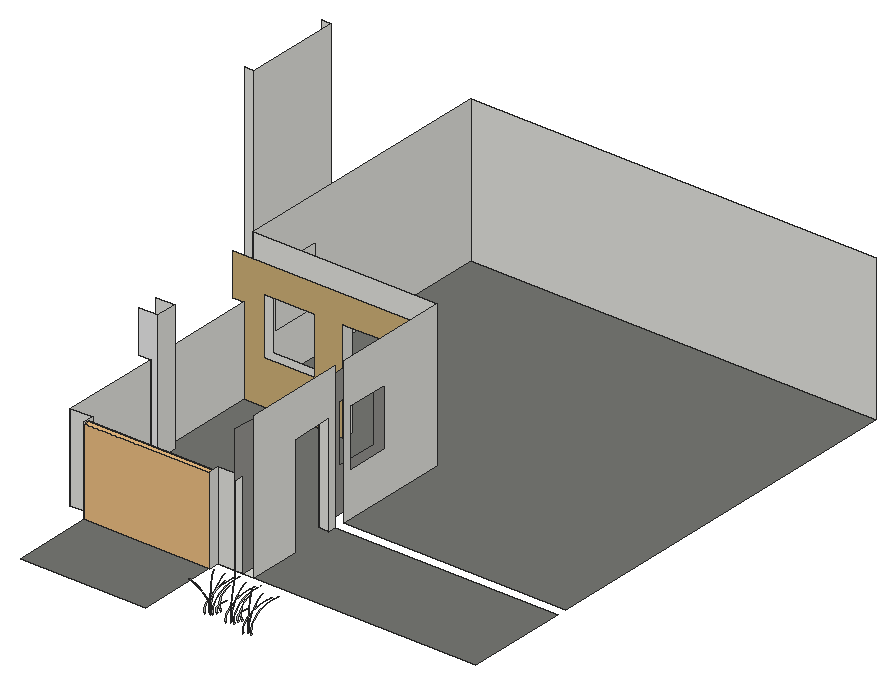
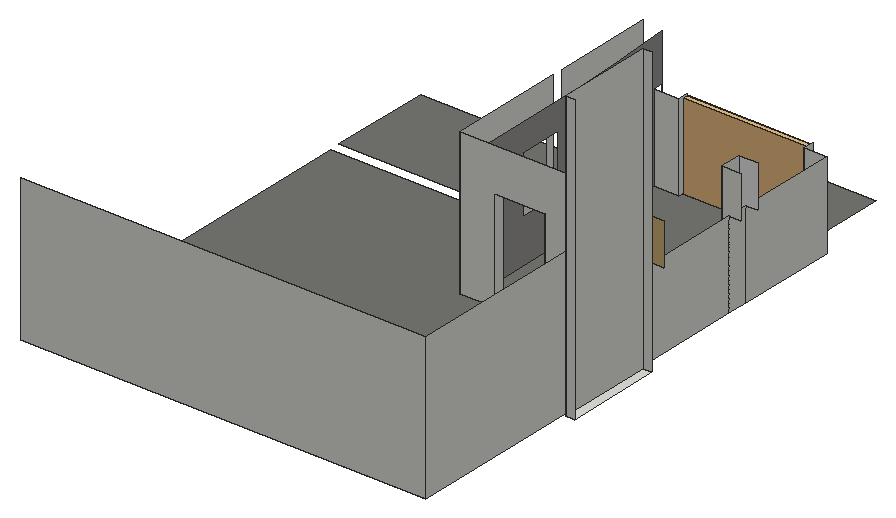
# SketchUp Ruby script. Lengths in inches.
U = 1.inch
M = Sketchup.active_model
def pt(a) = Geom::Point3d.new(a.map { |v| v * U })
def face(e, loops, mat)
  f = e.add_face(loops[0].map { |a| pt(a) })
  loops[1..].each { |l| e.add_face(l.map { |a| pt(a) }).erase! }
  f.material = f.back_material = mat if mat
  f
end
# faces: each face lists its corners as indices into pts; further lists are holes
def faces(e, pts, list, mat = nil) = list.each { |f| face(e, (f[0].is_a?(Array) ? f : [f]).map { |l| l.map { |i| pts[i] } }, mat) }
# xy, xz, yz: faces in a plane at the given z, y or x. An outline is a flat list of corners, or four numbers for a rectangle; further outlines are holes
def ring(l) = l.size == 4 ? [[l[0], l[1]], [l[2], l[1]], [l[2], l[3]], [l[0], l[3]]] : l.each_slice(2).to_a
def flat(e, list, mat, &to3) = list.each { |f| face(e, (f[0].is_a?(Array) ? f : [f]).map { |l| ring(l).map { |u, v| to3.(u, v) } }, mat) }
def xy(e, z, list, mat = nil) = flat(e, list, mat) { |x, y| [x, y, z] }
def xz(e, y, list, mat = nil) = flat(e, list, mat) { |x, z| [x, y, z] }
def yz(e, x, list, mat = nil) = flat(e, list, mat) { |y, z| [x, y, z] }
def lines(e, pts, list) = list.each { |a, b| e.add_line(pt(pts[a]), pt(pts[b])) }
# prism: a flat outline (further loops are holes) pulled along v
def prism(e, loops, v, mat = nil)
  f = face(e, loops, mat); d = Geom::Vector3d.new(v.map { |x| x * U })
  f.pushpull(f.normal.samedirection?(d) ? d.length : -d.length)
end
def box(e, o, s, mat = nil) = prism(e, [[o, [o[0] + s[0], o[1], o[2]], [o[0] + s[0], o[1] + s[1], o[2]], [o[0], o[1] + s[1], o[2]]]], [0, 0, s[2]], mat)
def at(x, y, z, deg = 0) = Geom::Transformation.translation(pt([x, y, z])) * Geom::Transformation.rotation(ORIGIN, Z_AXIS, deg.degrees)
def axes(o, x, y, z) = Geom::Transformation.new([*x, 0, *y, 0, *z, 0, *pt(o).to_a, 1])
def part(name) = M.definitions.add(name)
# library, detail: a bought-in or finely detailed component or shape, given as its bounding box
def library(name, o, s) = part(name).tap { |d| box(d.entities, o, s) }
def detail(e, o, s) = box(e.add_group.entities, o, s)
def put(e, d, t, mat = nil) = e.add_instance(d, t).tap { |i| i.material = mat if mat }
def group(e, t, mat = nil) = e.add_group.tap { |g| g.transformation = t; g.material = mat if mat }.entities
root = M.entities
M.materials.add("Metal_Seamed").color = [118, 119, 115]
M.materials.add("[Chipboard]").color = [205, 176, 119]
M.materials.add("[Granite Light Gray]").color = [149, 148, 144]
M.materials.add("white_wall").color = [233, 233, 233]
c1 = library("Merbau Gate Metal Frame",[0,0,0],[4.48,115.59,70.87])
xy(root,0,[[372.21,325.52,381.21,367.52],[229.21,408.6,235.21,426.23],[219.74,518.03,227.09,597.83]])
xy(root,0,[[247.49,251,351.06,251,351.06,317.12,351.48,317.12,351.48,325.52,372.21,325.52,372.21,367.52,381.21,367.52,381.21,325.52,565.21,325.52,565.21,409.52,381.21,409.52,381.21,403.52,372.21,403.52,372.21,505.52,352.83,505.52,352.83,514.52,381.21,514.52,381.21,418.52,565.21,418.52,565.21,739.58,229.21,739.58,229.21,514.52,310.83,514.52,310.83,505.52,229.21,505.52,229.21,426.23,235.21,426.23,235.21,408.6,229.21,408.6,229.21,325.52,247.49,325.52]],"Metal_Seamed")
xz(root,325.52,[[229.21,0,247.49,72],[351.48,0,372.21,72]])
xz(root,367.52,[[372.21,0,381.21,84]])
xz(root,403.52,[[372.21,0,381.21,84]])
xz(root,408.6,[[229.21,0,229.21,72,219.74,72,219.74,106.875,235.21,106.875,235.21,0]],"white_wall")
xz(root,426.23,[[229.21,0,235.21,0,235.21,106.875,219.74,106.875,219.74,72,229.21,72]])
xz(root,505.52,[[[229.21,0,310.83,0,310.83,84,352.83,84,352.83,0,372.21,0,372.21,106.875,219.74,106.875,219.74,72,229.21,72],[245.65,36,287.65,84]]],"[Chipboard]")
xz(root,514.52,[[[229.21,0,229.21,120,381.21,120,381.21,0,352.83,0,352.83,84,310.83,84,310.83,0],[245.65,36,287.65,84]]])
xz(root,518.03,[[219.74,0,227.09,237.3]])
xz(root,597.83,[[219.74,0,227.09,237.3]])
xz(root,739.58,[[229.21,0,565.21,120]])
yz(root,227.09,[[518.03,0,597.83,237.3]])
yz(root,229.21,[[325.52,0,408.6,72],[408.6,0,426.23,72],[426.23,0,505.52,72],[[514.52,0,739.58,120],[537.64,36,579.64,84]]])
yz(root,235.21,[[408.6,0,426.23,106.875]])
yz(root,247.49,[[317.12,0,325.52,72]])
yz(root,310.83,[[505.52,0,514.52,84]])
yz(root,351.48,[[317.12,0,325.52,72]])
yz(root,352.83,[[505.52,0,514.52,84]])
yz(root,372.21,[[317.12,0,317.13,0,317.13,72],[317.12,0,317.13,72,317.12,72],[[325.52,0,325.52,72,317.14,72,317.14,111,359.56,108.74,394.5,106.875,505.52,106.875,505.52,0,403.52,0,403.52,84,367.52,84,367.52,0],[424.52,36,460.52,84]]],"[Granite Light Gray]")
yz(root,381.21,[[325.52,0,367.52,0,367.52,84,403.52,84,403.52,0,409.52,0,409.52,120,325.52,120],[[418.52,0,514.52,120],[424.52,36,460.52,84]]])
g1 = group(root,at(386.9,271.43,0))
p = [[7.51,7.51,22.54],[6.3125,6.3125,20.88],[5.21,5.21,19.16],[4.21,4.21,17.39],[3.32,3.32,15.57],[2.52,2.52,13.71],
  [1.84,1.84,11.82],[1.27,1.27,9.89],[0.81,0.81,7.94],[0.46,0.46,5.97],[0.22,0.22,3.99],[0.1,0.1,2],
  [0.1,0.1,0],[0,0,2.01],[0.04,0.04,4.01],[0.21,0.21,6.01],[0.51,0.51,8],[0.95,0.95,9.97],
  [1.51,1.51,11.91],[2.21,2.21,13.81],[3.03,3.03,15.67],[3.98,3.98,17.48],[5.04,5.04,19.23],[6.22,6.22,20.92]]
faces(g1,p,[[0,1,2,3,4,5,6,7,8,9,10,11,12,13,14,15,16,17,18,19,20,21,22,23]])
g2 = group(root,at(390.32,270.24,0))
p = [[-0.93,0.35,0],[-0.41,0.16,0],[0,0,1.75],[-0.17,0.0625,3.51],[-0.91,0.34,5.24],[-2.21,0.83,6.89],
  [-4.03,1.52,8.42],[-6.34,2.39,9.8],[-9.0625,3.42,10.98],[-12.14,4.59,11.95],[-15.5,5.86,12.67],[-19.06,7.2,13.13],
  [-22.72,8.58,13.32],[-26.4,9.97,13.23],[-22.79,8.61,13.25],[-19.22,7.26,13],[-15.76,5.96,12.5],[-12.51,4.73,11.75],
  [-9.53,3.6,10.78],[-6.89,2.6,9.6],[-4.65,1.76,8.25],[-2.87,1.08,6.75],[-1.58,0.6,5.13],[-0.82,0.31,3.44],
  [-0.6,0.23,1.72]]
faces(g2,p,[[0,1,2,3,4,5,6,7,8,9,10,11,12,13,14,15,16,17,18,19,20,21,22,23,24]])
g3 = group(root,at(409.22,272.74,0))
p = [[5.08,5.08,9.0625],[4.15,4.15,8.49],[3.31,3.31,7.85],[2.57,2.57,7.18],[1.93,1.93,6.45],[1.41,1.41,5.7],
  [0.99,0.99,4.91],[0.7,0.7,4.1],[0.53,0.53,3.28],[0.48,0.48,2.45],[0.55,0.55,1.625],[0.75,0.75,0.8],
  [1.0625,1.0625,0],[0.65,0.65,0],[0.3,0.3,0.81],[0.08,0.08,1.65],[0,0,2.49],[0.06,0.06,3.34],
  [0.25,0.25,4.17],[0.58,0.58,4.99],[1.04,1.04,5.79],[1.62,1.62,6.54],[2.33,2.33,7.26],[3.14,3.14,7.92],
  [4.0625,4.0625,8.52]]
faces(g3,p,[[0,1,2,3,4,5,6,7,8,9,10,11,12,13,14,15,16,17,18,19,20,21,22,23,24]])
g4 = group(root,at(391.36,273.16,0))
p = [[5.08,5.08,9.0625],[4.15,4.15,8.49],[3.31,3.31,7.85],[2.57,2.57,7.18],[1.93,1.93,6.45],[1.41,1.41,5.7],
  [0.99,0.99,4.91],[0.7,0.7,4.1],[0.53,0.53,3.28],[0.48,0.48,2.45],[0.55,0.55,1.625],[0.75,0.75,0.8],
  [1.0625,1.0625,0],[0.65,0.65,0],[0.3,0.3,0.81],[0.08,0.08,1.65],[0,0,2.49],[0.06,0.06,3.34],
  [0.25,0.25,4.17],[0.58,0.58,4.99],[1.04,1.04,5.79],[1.62,1.62,6.54],[2.33,2.33,7.26],[3.14,3.14,7.92],
  [4.0625,4.0625,8.52]]
faces(g4,p,[[0,1,2,3,4,5,6,7,8,9,10,11,12,13,14,15,16,17,18,19,20,21,22,23,24]])
g5 = group(root,at(424.25,265.37,0))
p = [[-0.5,0.78,0],[-0.22,0.34,0],[0,0,2.37],[-0.09,0.14,4.75],[-0.49,0.76,7.08],[-1.2,1.84,9.32],
  [-2.1875,3.37,11.39],[-3.4375,5.29,13.25],[-4.92,7.57,14.85],[-6.59,10.14,16.15],[-8.41,12.95,17.13],[-10.34,15.92,17.75],
  [-12.32,18.97,18.01],[-14.32,22.05,17.89],[-12.36,19.03,17.91],[-10.42,16.05,17.58],[-8.55,13.16,16.9],[-6.78,10.45,15.89],
  [-5.17,7.96,14.58],[-3.73,5.75,12.99],[-2.52,3.88,11.15],[-1.55,2.39,9.125],[-0.86,1.32,6.94],[-0.44,0.68,4.66],
  [-0.33,0.5,2.33]]
faces(g5,p,[[0,1,2,3,4,5,6,7,8,9,10,11,12,13,14,15,16,17,18,19,20,21,22,23,24]])
g6 = group(root,at(421.55,263.18,0))
p = [[0.08,0.99,0],[0.03,0.44,0],[0,0,2.01],[0.01,0.18,4.04],[0.08,0.97,6.02],[0.19,2.35,7.92],
  [0.34,4.3,9.68],[0.53,6.75,11.26],[0.76,9.66,12.62],[1.02,12.94,13.73],[1.3,16.52,14.5625],[1.6,20.31,15.09],
  [1.91,24.21,15.31],[2.21,28.13,15.2],[1.91,24.29,15.22],[1.61,20.48,14.94],[1.32,16.8,14.37],[1.05,13.33,13.51],
  [0.8,10.15,12.39],[0.58,7.34,11.04],[0.39,4.95,9.48],[0.24,3.05,7.75],[0.13,1.68,5.9],[0.07,0.87,3.96],
  [0.05,0.64,1.98]]
faces(g6,p,[[0,1,2,3,4,5,6,7,8,9,10,11,12,13,14,15,16,17,18,19,20,21,22,23,24]])
g7 = group(root,at(427.01,264.89,0))
p = [[0.07,0.92,0],[0.03,0.41,0],[0,0,2.37],[0.01,0.17,4.75],[0.07,0.9,7.08],[0.17,2.19,9.32],
  [0.32,4,11.39],[0.5,6.29,13.25],[0.71,9,14.85],[0.95,12.06,16.15],[1.21,15.39,17.13],[1.49,18.92,17.75],
  [1.78,22.55,18.01],[2.0625,26.21,17.89],[1.78,22.625,17.91],[1.5,19.08,17.58],[1.23,15.65,16.9],[0.98,12.42,15.89],
  [0.74,9.46,14.58],[0.54,6.84,12.99],[0.36,4.61,11.15],[0.22,2.84,9.125],[0.125,1.57,6.94],[0.0625,0.8125,4.66],
  [0.05,0.59,2.33]]
faces(g7,p,[[0,1,2,3,4,5,6,7,8,9,10,11,12,13,14,15,16,17,18,19,20,21,22,23,24]])
g8 = group(root,at(409.57,275.82,0))
p = [[5.08,5.08,18.42],[4.15,4.15,17.25],[3.31,3.31,15.97],[2.57,2.57,14.59],[1.93,1.93,13.12],[1.41,1.41,11.58],
  [0.99,0.99,9.98],[0.7,0.7,8.34],[0.53,0.53,6.67],[0.48,0.48,4.99],[0.55,0.55,3.3],[0.75,0.75,1.63],
  [1.0625,1.0625,0],[0.65,0.65,0],[0.3,0.3,1.66],[0.08,0.08,3.35],[0,0,5.07],[0.06,0.06,6.79],
  [0.25,0.25,8.49],[0.58,0.58,10.15],[1.04,1.04,11.76],[1.62,1.62,13.3],[2.33,2.33,14.75],[3.14,3.14,16.1],
  [4.0625,4.0625,17.33]]
faces(g8,p,[[0,1,2,3,4,5,6,7,8,9,10,11,12,13,14,15,16,17,18,19,20,21,22,23,24]])
g9 = group(root,at(391.7,276.23,0))
p = [[5.08,5.08,18.42],[4.15,4.15,17.25],[3.31,3.31,15.97],[2.57,2.57,14.59],[1.93,1.93,13.12],[1.41,1.41,11.58],
  [0.99,0.99,9.98],[0.7,0.7,8.34],[0.53,0.53,6.67],[0.48,0.48,4.99],[0.55,0.55,3.3],[0.75,0.75,1.63],
  [1.0625,1.0625,0],[0.65,0.65,0],[0.3,0.3,1.66],[0.08,0.08,3.35],[0,0,5.07],[0.06,0.06,6.79],
  [0.25,0.25,8.49],[0.58,0.58,10.15],[1.04,1.04,11.76],[1.62,1.62,13.3],[2.33,2.33,14.75],[3.14,3.14,16.1],
  [4.0625,4.0625,17.33]]
faces(g9,p,[[0,1,2,3,4,5,6,7,8,9,10,11,12,13,14,15,16,17,18,19,20,21,22,23,24]])
g10 = group(root,at(423.97,266.21,0))
p = [[-0.27,0.88,0],[-0.12,0.39,0],[0,0,2.0625],[-0.05,0.16,4.13],[-0.26,0.87,6.16],[-0.64,2.1,8.1],
  [-1.17,3.84,9.91],[-1.84,6.03,11.52],[-2.64,8.63,12.92],[-3.54,11.5625,14.05],[-4.51,14.76,14.9],[-5.55,18.15,15.45],
  [-6.61,21.64,15.67],[-7.69,25.14,15.5625],[-6.63,21.7,15.58],[-5.59,18.3,15.29],[-4.59,15.01,14.71],[-3.64,11.91,13.83],
  [-2.77,9.07,12.68],[-2,6.56,11.3],[-1.35,4.43,9.7],[-0.83,2.73,7.9375],[-0.46,1.5,6.04],[-0.24,0.78,4.05],
  [-0.17,0.57,2.02]]
faces(g10,p,[[0,1,2,3,4,5,6,7,8,9,10,11,12,13,14,15,16,17,18,19,20,21,22,23,24]])
g11 = group(root,at(406.55,269.72,0))
p = [[-0.5,0.78,0],[-0.22,0.34,0],[0,0,2.37],[-0.09,0.14,4.75],[-0.49,0.76,7.08],[-1.2,1.84,9.32],
  [-2.1875,3.37,11.39],[-3.4375,5.29,13.25],[-4.92,7.57,14.85],[-6.59,10.14,16.15],[-8.41,12.95,17.13],[-10.34,15.92,17.75],
  [-12.32,18.97,18.01],[-14.32,22.05,17.89],[-12.36,19.03,17.91],[-10.42,16.05,17.58],[-8.55,13.16,16.9],[-6.78,10.45,15.89],
  [-5.17,7.96,14.58],[-3.73,5.75,12.99],[-2.52,3.88,11.15],[-1.55,2.39,9.125],[-0.86,1.32,6.94],[-0.44,0.68,4.66],
  [-0.33,0.5,2.33]]
faces(g11,p,[[0,1,2,3,4,5,6,7,8,9,10,11,12,13,14,15,16,17,18,19,20,21,22,23,24]])
g12 = group(root,at(388.68,270.13,0))
p = [[-0.5,0.78,0],[-0.22,0.34,0],[0,0,2.37],[-0.09,0.14,4.75],[-0.49,0.76,7.08],[-1.2,1.84,9.32],
  [-2.1875,3.37,11.39],[-3.4375,5.29,13.25],[-4.92,7.57,14.85],[-6.59,10.14,16.15],[-8.41,12.95,17.13],[-10.34,15.92,17.75],
  [-12.32,18.97,18.01],[-14.32,22.05,17.89],[-12.36,19.03,17.91],[-10.42,16.05,17.58],[-8.55,13.16,16.9],[-6.78,10.45,15.89],
  [-5.17,7.96,14.58],[-3.73,5.75,12.99],[-2.52,3.88,11.15],[-1.55,2.39,9.125],[-0.86,1.32,6.94],[-0.44,0.68,4.66],
  [-0.33,0.5,2.33]]
faces(g12,p,[[0,1,2,3,4,5,6,7,8,9,10,11,12,13,14,15,16,17,18,19,20,21,22,23,24]])
g13 = group(root,at(403.84,267.53,0))
p = [[0.08,0.99,0],[0.03,0.44,0],[0,0,2.01],[0.01,0.18,4.04],[0.08,0.97,6.02],[0.19,2.35,7.92],
  [0.34,4.3,9.68],[0.53,6.75,11.26],[0.76,9.66,12.62],[1.02,12.94,13.73],[1.3,16.52,14.5625],[1.6,20.31,15.09],
  [1.91,24.21,15.31],[2.21,28.13,15.2],[1.91,24.29,15.22],[1.61,20.48,14.94],[1.32,16.8,14.37],[1.05,13.33,13.51],
  [0.8,10.15,12.39],[0.58,7.34,11.04],[0.39,4.95,9.48],[0.24,3.05,7.75],[0.13,1.68,5.9],[0.07,0.87,3.96],
  [0.05,0.64,1.98]]
faces(g13,p,[[0,1,2,3,4,5,6,7,8,9,10,11,12,13,14,15,16,17,18,19,20,21,22,23,24]])
g14 = group(root,at(385.98,267.95,0))
p = [[0.08,0.99,0],[0.03,0.44,0],[0,0,2.01],[0.01,0.18,4.04],[0.08,0.97,6.02],[0.19,2.35,7.92],
  [0.34,4.3,9.68],[0.53,6.75,11.26],[0.76,9.66,12.62],[1.02,12.94,13.73],[1.3,16.52,14.5625],[1.6,20.31,15.09],
  [1.91,24.21,15.31],[2.21,28.13,15.2],[1.91,24.29,15.22],[1.61,20.48,14.94],[1.32,16.8,14.37],[1.05,13.33,13.51],
  [0.8,10.15,12.39],[0.58,7.34,11.04],[0.39,4.95,9.48],[0.24,3.05,7.75],[0.13,1.68,5.9],[0.07,0.87,3.96],
  [0.05,0.64,1.98]]
faces(g14,p,[[0,1,2,3,4,5,6,7,8,9,10,11,12,13,14,15,16,17,18,19,20,21,22,23,24]])
g15 = group(root,at(409.3,269.24,0))
p = [[0.07,0.92,0],[0.03,0.41,0],[0,0,2.37],[0.01,0.17,4.75],[0.07,0.9,7.08],[0.17,2.19,9.32],
  [0.32,4,11.39],[0.5,6.29,13.25],[0.71,9,14.85],[0.95,12.06,16.15],[1.21,15.39,17.13],[1.49,18.92,17.75],
  [1.78,22.55,18.01],[2.0625,26.21,17.89],[1.78,22.625,17.91],[1.5,19.08,17.58],[1.23,15.65,16.9],[0.98,12.42,15.89],
  [0.74,9.46,14.58],[0.54,6.84,12.99],[0.36,4.61,11.15],[0.22,2.84,9.125],[0.125,1.57,6.94],[0.0625,0.8125,4.66],
  [0.05,0.59,2.33]]
faces(g15,p,[[0,1,2,3,4,5,6,7,8,9,10,11,12,13,14,15,16,17,18,19,20,21,22,23,24]])
g16 = group(root,at(391.4375,269.66,0))
p = [[0.07,0.92,0],[0.03,0.41,0],[0,0,2.37],[0.01,0.17,4.75],[0.07,0.9,7.08],[0.17,2.19,9.32],
  [0.32,4,11.39],[0.5,6.29,13.25],[0.71,9,14.85],[0.95,12.06,16.15],[1.21,15.39,17.13],[1.49,18.92,17.75],
  [1.78,22.55,18.01],[2.0625,26.21,17.89],[1.78,22.625,17.91],[1.5,19.08,17.58],[1.23,15.65,16.9],[0.98,12.42,15.89],
  [0.74,9.46,14.58],[0.54,6.84,12.99],[0.36,4.61,11.15],[0.22,2.84,9.125],[0.125,1.57,6.94],[0.0625,0.8125,4.66],
  [0.05,0.59,2.33]]
faces(g16,p,[[0,1,2,3,4,5,6,7,8,9,10,11,12,13,14,15,16,17,18,19,20,21,22,23,24]])
g17 = group(root,at(406.26,270.56,0))
p = [[-0.27,0.88,0],[-0.12,0.39,0],[0,0,2.0625],[-0.05,0.16,4.13],[-0.26,0.87,6.16],[-0.64,2.1,8.1],
  [-1.17,3.84,9.91],[-1.84,6.03,11.52],[-2.64,8.63,12.92],[-3.54,11.5625,14.05],[-4.51,14.76,14.9],[-5.55,18.15,15.45],
  [-6.61,21.64,15.67],[-7.69,25.14,15.5625],[-6.63,21.7,15.58],[-5.59,18.3,15.29],[-4.59,15.01,14.71],[-3.64,11.91,13.83],
  [-2.77,9.07,12.68],[-2,6.56,11.3],[-1.35,4.43,9.7],[-0.83,2.73,7.9375],[-0.46,1.5,6.04],[-0.24,0.78,4.05],
  [-0.17,0.57,2.02]]
faces(g17,p,[[0,1,2,3,4,5,6,7,8,9,10,11,12,13,14,15,16,17,18,19,20,21,22,23,24]])
g18 = group(root,at(388.4,270.98,0))
p = [[-0.27,0.88,0],[-0.12,0.39,0],[0,0,2.0625],[-0.05,0.16,4.13],[-0.26,0.87,6.16],[-0.64,2.1,8.1],
  [-1.17,3.84,9.91],[-1.84,6.03,11.52],[-2.64,8.63,12.92],[-3.54,11.5625,14.05],[-4.51,14.76,14.9],[-5.55,18.15,15.45],
  [-6.61,21.64,15.67],[-7.69,25.14,15.5625],[-6.63,21.7,15.58],[-5.59,18.3,15.29],[-4.59,15.01,14.71],[-3.64,11.91,13.83],
  [-2.77,9.07,12.68],[-2,6.56,11.3],[-1.35,4.43,9.7],[-0.83,2.73,7.9375],[-0.46,1.5,6.04],[-0.24,0.78,4.05],
  [-0.17,0.57,2.02]]
faces(g18,p,[[0,1,2,3,4,5,6,7,8,9,10,11,12,13,14,15,16,17,18,19,20,21,22,23,24]])
put(root,c1,axes([351.48,317.12,0],[0,1,0],[-0.89957,0,0],[0,0,1]))
